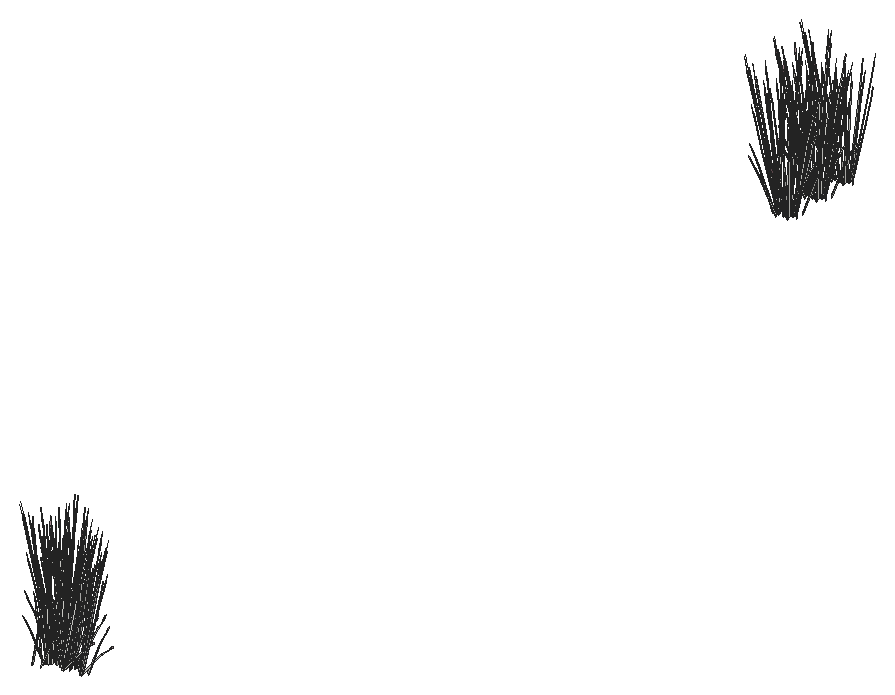
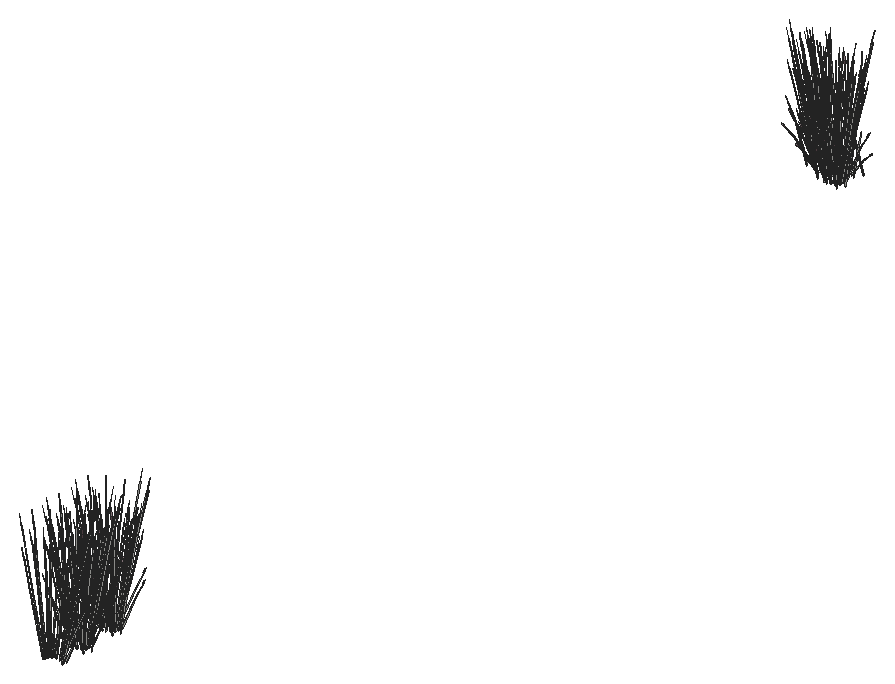
# SketchUp Ruby script. Lengths in inches.
U = 1.inch
M = Sketchup.active_model
def pt(a) = Geom::Point3d.new(a.map { |v| v * U })
def face(e, loops, mat)
  f = e.add_face(loops[0].map { |a| pt(a) })
  loops[1..].each { |l| e.add_face(l.map { |a| pt(a) }).erase! }
  f.material = f.back_material = mat if mat
  f
end
# faces: each face lists its corners as indices into pts; further lists are holes
def faces(e, pts, list, mat = nil) = list.each { |f| face(e, (f[0].is_a?(Array) ? f : [f]).map { |l| l.map { |i| pts[i] } }, mat) }
# xy, xz, yz: faces in a plane at the given z, y or x. An outline is a flat list of corners, or four numbers for a rectangle; further outlines are holes
def ring(l) = l.size == 4 ? [[l[0], l[1]], [l[2], l[1]], [l[2], l[3]], [l[0], l[3]]] : l.each_slice(2).to_a
def flat(e, list, mat, &to3) = list.each { |f| face(e, (f[0].is_a?(Array) ? f : [f]).map { |l| ring(l).map { |u, v| to3.(u, v) } }, mat) }
def xy(e, z, list, mat = nil) = flat(e, list, mat) { |x, y| [x, y, z] }
def xz(e, y, list, mat = nil) = flat(e, list, mat) { |x, z| [x, y, z] }
def yz(e, x, list, mat = nil) = flat(e, list, mat) { |y, z| [x, y, z] }
def lines(e, pts, list) = list.each { |a, b| e.add_line(pt(pts[a]), pt(pts[b])) }
# prism: a flat outline (further loops are holes) pulled along v
def prism(e, loops, v, mat = nil)
  f = face(e, loops, mat); d = Geom::Vector3d.new(v.map { |x| x * U })
  f.pushpull(f.normal.samedirection?(d) ? d.length : -d.length)
end
def box(e, o, s, mat = nil) = prism(e, [[o, [o[0] + s[0], o[1], o[2]], [o[0] + s[0], o[1] + s[1], o[2]], [o[0], o[1] + s[1], o[2]]]], [0, 0, s[2]], mat)
def at(x, y, z, deg = 0) = Geom::Transformation.translation(pt([x, y, z])) * Geom::Transformation.rotation(ORIGIN, Z_AXIS, deg.degrees)
def axes(o, x, y, z) = Geom::Transformation.new([*x, 0, *y, 0, *z, 0, *pt(o).to_a, 1])
def part(name) = M.definitions.add(name)
# library, detail: a bought-in or finely detailed component or shape, given as its bounding box
def library(name, o, s) = part(name).tap { |d| box(d.entities, o, s) }
def detail(e, o, s) = box(e.add_group.entities, o, s)
def put(e, d, t, mat = nil) = e.add_instance(d, t).tap { |i| i.material = mat if mat }
def group(e, t, mat = nil) = e.add_group.tap { |g| g.transformation = t; g.material = mat if mat }.entities
root = M.entities
M.materials.add("LightPink_Translucent").color = [144, 107, 117]
M.materials["LightPink_Translucent"].alpha = 0.75
c1 = part("blade")
p = [[2.15,0.21,22],[0,0.17,0],[0.09,0.45,0],[2.18,0.31,22],[2.29,0.31,22],[0.38,0.45,0],
  [2.48,0.24,33],[2.49,0.24,33],[2.48,0.22,33]]
faces(c1.entities,p,[[0,1,2,3],[4,5,2,3],[6,3,4,7],[8,0,3,6]])
c2 = part("seeds")
p = [[0.3,-0.1,1.38],[-0.01,-0.03,1.59],[-0.01,-0.03,0.03],[0.14,-0.07,-0.07],[0.29,-0.03,3],[0.15,0.01,3.11]]
faces(c2.entities,p,[[0,1,2,3],[1,0,4,5]],"LightPink_Translucent")
c3 = part("blade with seeds")
put(c3.entities,c1,at(0,0,0))
put(c3.entities,c2,axes([2.4,0.25,30.99],[1.5799,-0.05474,1.17369],[-0.12525,1.92788,0.29478],[-0.07173,-0.02425,1.56792]))
put(root,c3,axes([334.01,30.38,52.18],[0.22948,-0.24822,0.05682],[0.32679,0.14452,0.44729],[-0.10565,-0.07958,0.68204]))
put(root,c3,axes([341.83,29.48,52.46],[-0.41962,-0.10901,0.31292],[0.12239,-0.31802,-0.40398],[0.16894,-0.02916,0.77298]))
put(root,c3,axes([337.4375,28.9,52.18],[0.14265,-0.35629,0.42415],[0.46898,0.12183,0.34973],[-0.18443,0.02141,0.87768]))
put(root,c3,axes([331.05,26.46,52.16],[0.05728,-0.02359,1.56736],[0.47345,0.15692,-0.1481],[-0.01113,0.13066,0.27737]))
put(root,c3,axes([335.14,30.62,52.46],[-0.15222,0.30049,0.31292],[-0.44409,-0.08764,-0.40398],[-0.04072,-0.12098,0.77298]))
put(root,c3,axes([337.4,28.8,52.18],[-0.18545,-0.26643,0.05682],[0.33817,-0.13041,0.44729],[-0.14907,0.02573,0.68204]))
put(root,c3,axes([336.28,30.75,52.18],[0.35954,0.26661,0.42415],[-0.38183,0.22994,0.34973],[0.06632,-0.12508,0.87768]))
put(root,c3,axes([334.11,30.36,52.8],[-0.33698,0.3746,-0.12034],[-0.48801,-0.21581,-0.66795],[-0.16964,-0.10584,1.01494]))
put(root,c3,axes([336.41,30.77,52.18],[0.41493,0.01821,0.05682],[-0.01138,0.27493,0.44729],[0.04342,-0.10531,0.68204]))
put(root,c3,axes([338.86,29.54,52.16],[-0.04566,-0.03421,1.56736],[0.09987,-0.36669,-0.1481],[0.17984,-0.02343,0.27737]))
put(root,c3,axes([336.1,30.96,52.46],[-0.34164,0.20573,0.31292],[-0.3234,-0.23491,-0.40398],[0.04921,-0.11936,0.77298]))
put(root,c3,axes([332.92,28.05,52.17],[-0.08245,0.05073,1.54581],[0.00701,0.37067,-0.24447],[-0.18899,0.0482,0.12397]))
put(root,c3,axes([333.14,26.625,52.17],[0.064,0.06292,1.54581],[0.51651,0.02472,-0.24447],[0.05194,0.13877,0.12397]))
put(root,c3,axes([337.2,29.07,52.46],[-0.28729,-0.24465,0.31292],[0.32804,-0.23159,-0.40398],[0.16667,0.03524,0.77298]))
put(root,c3,axes([334.08,30.67,52.46],[0.07798,0.31474,0.31292],[-0.44579,0.08311,-0.40398],[-0.11974,-0.09019,0.77298]))
put(root,c3,axes([342.21,29.58,52.18],[0.18545,0.26643,0.05682],[-0.33817,0.13041,0.44729],[0.14907,-0.02573,0.68204]))
put(root,c3,axes([332.74,30.875,52.5],[0.41698,-0.28837,0.47505],[0.35962,0.30624,0.3917],[-0.19563,-0.05319,0.983]))
put(root,c3,axes([338.07,31.53,52.16],[-0.06595,-0.00297,1.56736],[-0.27386,-0.31799,-0.1481],[0.10998,-0.10455,0.27737]))
put(root,c3,axes([342.18,29.48,52.18],[-0.14265,0.35629,0.42415],[-0.46898,-0.12183,0.34973],[0.18443,-0.02141,0.87768]))
put(root,c3,axes([337.73,28.99,52.17],[0.10831,-0.00661,1.54581],[0.29709,-0.30358,-0.24447],[0.19266,0.04007,0.12397]))
put(root,c3,axes([337.78,28.9,52.46],[0.41962,0.10901,0.31292],[-0.12239,0.31802,-0.40398],[-0.16894,0.02916,0.77298]))
put(root,c3,axes([333.39,28.69,52.18],[-0.12522,-0.35963,0.42415],[0.49122,-0.06241,0.34973],[-0.14477,0.08458,0.87768]))
put(root,c3,axes([333.3,28.62,52.18],[-0.34663,-0.16434,0.05682],[0.20181,-0.23402,0.44729],[-0.11113,0.07566,0.68204]))
put(root,c3,axes([332.93,30.87,52.18],[0.02542,-0.29714,0.05682],[0.38391,0.00815,0.44729],[-0.14706,-0.03109,0.68204]))
put(root,c3,axes([336.69,31.59,52.46],[-0.43951,0.05584,0.31292],[-0.11606,-0.31924,-0.40398],[0.12595,-0.08575,0.77298]))
put(root,c3,axes([343.02,30.64,52.16],[-0.04566,-0.03421,1.56736],[0.09987,-0.36669,-0.1481],[0.17984,-0.02343,0.27737]))
put(root,c3,axes([333.7,28.57,52.46],[0.43951,-0.05584,0.31292],[0.11606,0.31924,-0.40398],[-0.12595,0.08575,0.77298]))
put(root,c3,axes([332,28.43,52.16],[0.06444,0.01048,1.56736],[0.19934,0.34525,-0.1481],[-0.13191,0.09062,0.27737]))
put(root,c3,axes([337.08,29.15,52.17],[-0.08245,0.05073,1.54581],[0.00701,0.37067,-0.24447],[-0.18899,0.0482,0.12397]))
put(root,c3,axes([337.46,29.29,52.18],[-0.02542,0.29714,0.05682],[-0.38391,-0.00815,0.44729],[0.14706,0.03109,0.68204]))
put(root,c3,axes([337.5,29.2,52.18],[-0.3723,0.25748,0.42415],[-0.32109,-0.27343,0.34973],[0.17467,0.04749,0.87768]))
put(root,c3,axes([341.36,30.17,52.46],[-0.28729,-0.24465,0.31292],[0.32804,-0.23159,-0.40398],[0.16667,0.03524,0.77298]))
put(root,c3,axes([337.09,31.54,52.18],[0.34663,0.16434,0.05682],[-0.20181,0.23402,0.44729],[0.11113,-0.07566,0.68204]))
put(root,c3,axes([337,31.47,52.18],[0.12522,0.35963,0.42415],[-0.49122,0.06241,0.34973],[0.14477,-0.08458,0.87768]))
put(root,c3,axes([332.7,29.48,52.99],[0.44556,0.1043,-0.05733],[-0.13706,0.32103,-0.25992],[-0.07288,0.04874,0.85731]))
put(root,c3,axes([336.3125,29.5,52.46],[-0.07798,-0.31474,0.31292],[0.44579,-0.08311,-0.40398],[0.11974,0.09019,0.77298]))
put(root,c3,axes([332.4,30.48,52.16],[0.03743,0.039,1.56736],[-0.18045,0.35054,-0.1481],[-0.18276,0.00254,0.27737]))
put(root,c3,axes([341.88,30.08,52.17],[0.10831,-0.00661,1.54581],[0.29709,-0.30358,-0.24447],[0.19266,0.04007,0.12397]))
put(root,c3,axes([337.55,29.79,52.18],[-0.12522,-0.35963,0.42415],[0.49122,-0.06241,0.34973],[-0.14477,0.08458,0.87768]))
put(root,c3,axes([337.45,29.72,52.18],[-0.34663,-0.16434,0.05682],[0.20181,-0.23402,0.44729],[-0.11113,0.07566,0.68204]))
put(root,c3,axes([333.1875,31.09,52.46],[0.28729,0.24465,0.31292],[-0.32804,0.23159,-0.40398],[-0.16667,-0.03524,0.77298]))
put(root,c3,axes([334.29,29.21,52.46],[0.34164,-0.20573,0.31292],[0.3234,0.23491,-0.40398],[-0.04921,0.11936,0.77298]))
put(root,c3,axes([335.88,29.9375,52.16],[0.00149,-0.04731,1.56736],[0.4327,-0.20872,-0.1481],[0.1503,0.0745,0.27737]))
put(root,c3,axes([337.85,29.67,52.46],[0.43951,-0.05584,0.31292],[0.11606,0.31924,-0.40398],[-0.12595,0.08575,0.77298]))
put(root,c3,axes([333.98,29.39,52.18],[-0.41493,-0.01821,0.05682],[0.01138,-0.27493,0.44729],[-0.04342,0.10531,0.68204]))
put(root,c3,axes([336.16,29.52,52.16],[0.06444,0.01048,1.56736],[0.19934,0.34525,-0.1481],[-0.13191,0.09062,0.27737]))
put(root,c3,axes([334.11,29.42,52.18],[-0.35954,-0.26661,0.42415],[0.38183,-0.22994,0.34973],[-0.06632,0.12508,0.87768]))
put(root,c3,axes([335.25,29.55,52.46],[0.15222,-0.30049,0.31292],[0.44409,0.08764,-0.40398],[0.04072,0.12098,0.77298]))
put(root,c3,axes([341.62,30.39,52.18],[-0.02542,0.29714,0.05682],[-0.38391,-0.00815,0.44729],[0.14706,0.03109,0.68204]))
put(root,c3,axes([341.65,30.29,52.18],[-0.3723,0.25748,0.42415],[-0.32109,-0.27343,0.34973],[0.17467,0.04749,0.87768]))
put(root,c3,axes([336.38,29.78,52.18],[-0.22948,0.24822,0.05682],[-0.32679,-0.14452,0.44729],[0.10565,0.07958,0.68204]))
put(root,c3,axes([335.84,30.62,52.99],[0.34892,-0.22417,-0.05733],[0.3197,0.24551,-0.25992],[0.02251,0.06957,0.85731]))
put(root,c3,axes([336.76,32.36,52.46],[-0.41962,-0.10901,0.31292],[0.12239,-0.31802,-0.40398],[0.16894,-0.02916,0.77298]))
put(root,c3,axes([336.48,29.71,52.18],[-0.5022,0.08967,0.42415],[-0.08716,-0.35177,0.34973],[0.11811,0.10367,0.87768]))
put(root,c3,axes([336.85,30.57,52.99],[0.44556,0.1043,-0.05733],[-0.13706,0.32103,-0.25992],[-0.07288,0.04874,0.85731]))
put(root,c3,axes([332.37,31.78,52.18],[0.14265,-0.35629,0.42415],[0.46898,0.12183,0.34973],[-0.18443,0.02141,0.87768]))
put(root,c3,axes([332.34,31.68,52.18],[-0.18545,-0.26643,0.05682],[0.33817,-0.13041,0.44729],[-0.14907,0.02573,0.68204]))
put(root,c3,axes([340.47,30.59,52.46],[-0.07798,-0.31474,0.31292],[0.44579,-0.08311,-0.40398],[0.11974,0.09019,0.77298]))
put(root,c3,axes([335.11,29.82,52.18],[-0.37205,0.1328,0.05682],[-0.18211,-0.24217,0.44729],[0.03593,0.10675,0.68204]))
put(root,c3,axes([332.93,29.4375,52.17],[-0.01255,0.07733,1.54581],[0.35618,0.269,-0.24447],[-0.09325,0.12721,0.12397]))
put(root,c3,axes([334.07,29.26,52.77],[0.55492,0.01936,-0.11927],[-0.01517,0.36657,-0.66198],[-0.03855,0.14118,1.00587]))
put(root,c3,axes([335.24,29.79,52.47],[-0.49753,-0.10215,0.47081],[0.17013,-0.33585,0.3882],[0.0299,0.13207,0.97422]))
put(root,c3,axes([338.45,30.3,52.46],[0.34164,-0.20573,0.31292],[0.3234,0.23491,-0.40398],[-0.04921,0.11936,0.77298]))
put(root,c3,axes([340.04,31.03,52.16],[0.00149,-0.04731,1.56736],[0.4327,-0.20872,-0.1481],[0.1503,0.0745,0.27737]))
put(root,c3,axes([338.14,30.49,52.18],[-0.41493,-0.01821,0.05682],[0.01138,-0.27493,0.44729],[-0.04342,0.10531,0.68204]))
put(root,c3,axes([338.27,30.51,52.18],[-0.35954,-0.26661,0.42415],[0.38183,-0.22994,0.34973],[-0.06632,0.12508,0.87768]))
put(root,c3,axes([337.14,32.46,52.18],[0.18545,0.26643,0.05682],[-0.33817,0.13041,0.44729],[0.14907,-0.02573,0.68204]))
put(root,c3,axes([339.4,30.64,52.46],[0.15222,-0.30049,0.31292],[0.44409,0.08764,-0.40398],[0.04072,0.12098,0.77298]))
put(root,c3,axes([337.11,32.36,52.18],[-0.14265,0.35629,0.42415],[-0.46898,-0.12183,0.34973],[0.18443,-0.02141,0.87768]))
put(root,c3,axes([332.72,31.78,52.46],[0.41962,0.10901,0.31292],[-0.12239,0.31802,-0.40398],[-0.16894,0.02916,0.77298]))
put(root,c3,axes([332.89,30.23,52.16],[0.05728,-0.02359,1.56736],[0.47345,0.15692,-0.1481],[-0.01113,0.13066,0.27737]))
put(root,c3,axes([340.54,30.875,52.18],[-0.22948,0.24822,0.05682],[-0.32679,-0.14452,0.44729],[0.10565,0.07958,0.68204]))
put(root,c3,axes([340,31.71,52.99],[0.34892,-0.22417,-0.05733],[0.3197,0.24551,-0.25992],[0.02251,0.06957,0.85731]))
put(root,c3,axes([340.64,30.81,52.18],[-0.5022,0.08967,0.42415],[-0.08716,-0.35177,0.34973],[0.11811,0.10367,0.87768]))
put(root,c3,axes([337.95,33.52,52.16],[-0.04566,-0.03421,1.56736],[0.09987,-0.36669,-0.1481],[0.17984,-0.02343,0.27737]))
put(root,c3,axes([339.27,30.91,52.18],[-0.37205,0.1328,0.05682],[-0.18211,-0.24217,0.44729],[0.03593,0.10675,0.68204]))
put(root,c3,axes([337.09,30.53,52.17],[-0.01255,0.07733,1.54581],[0.35618,0.269,-0.24447],[-0.09325,0.12721,0.12397]))
put(root,c3,axes([334.98,30.4,52.17],[0.064,0.06292,1.54581],[0.51651,0.02472,-0.24447],[0.05194,0.13877,0.12397]))
put(root,c3,axes([338.23,30.36,52.77],[0.55492,0.01936,-0.11927],[-0.01517,0.36657,-0.66198],[-0.03855,0.14118,1.00587]))
put(root,c3,axes([339.4,30.89,52.47],[-0.49753,-0.10215,0.47081],[0.17013,-0.33585,0.3882],[0.0299,0.13207,0.97422]))
put(root,c3,axes([336.29,33.04,52.46],[-0.28729,-0.24465,0.31292],[0.32804,-0.23159,-0.40398],[0.16667,0.03524,0.77298]))
put(root,c3,axes([332.48,32.66,52.18],[-0.12522,-0.35963,0.42415],[0.49122,-0.06241,0.34973],[-0.14477,0.08458,0.87768]))
put(root,c3,axes([332.39,32.59,52.18],[-0.34663,-0.16434,0.05682],[0.20181,-0.23402,0.44729],[-0.11113,0.07566,0.68204]))
put(root,c3,axes([337.05,31.33,52.16],[0.05728,-0.02359,1.56736],[0.47345,0.15692,-0.1481],[-0.01113,0.13066,0.27737]))
put(root,c3,axes([332.79,32.54,52.46],[0.43951,-0.05584,0.31292],[0.11606,0.31924,-0.40398],[-0.12595,0.08575,0.77298]))
put(root,c3,axes([339.14,31.49,52.17],[0.064,0.06292,1.54581],[0.51651,0.02472,-0.24447],[0.05194,0.13877,0.12397]))
put(root,c3,axes([331.09,32.4,52.16],[0.06444,0.01048,1.56736],[0.19934,0.34525,-0.1481],[-0.13191,0.09062,0.27737]))
put(root,c3,axes([336.55,33.27,52.18],[-0.02542,0.29714,0.05682],[-0.38391,-0.00815,0.44729],[0.14706,0.03109,0.68204]))
put(root,c3,axes([336.59,33.17,52.18],[-0.3723,0.25748,0.42415],[-0.32109,-0.27343,0.34973],[0.17467,0.04749,0.87768]))
put(root,c3,axes([331.79,33.45,52.99],[0.44556,0.1043,-0.05733],[-0.13706,0.32103,-0.25992],[-0.07288,0.04874,0.85731]))
put(root,c3,axes([335.4,33.47,52.46],[-0.07798,-0.31474,0.31292],[0.44579,-0.08311,-0.40398],[0.11974,0.09019,0.77298]))
put(root,c3,axes([333.38,33.18,52.46],[0.34164,-0.20573,0.31292],[0.3234,0.23491,-0.40398],[-0.04921,0.11936,0.77298]))
put(root,c3,axes([334.97,33.91,52.16],[0.00149,-0.04731,1.56736],[0.4327,-0.20872,-0.1481],[0.1503,0.0745,0.27737]))
put(root,c3,axes([333.07,33.37,52.18],[-0.41493,-0.01821,0.05682],[0.01138,-0.27493,0.44729],[-0.04342,0.10531,0.68204]))
put(root,c3,axes([333.2,33.39,52.18],[-0.35954,-0.26661,0.42415],[0.38183,-0.22994,0.34973],[-0.06632,0.12508,0.87768]))
put(root,c3,axes([334.34,33.52,52.46],[0.15222,-0.30049,0.31292],[0.44409,0.08764,-0.40398],[0.04072,0.12098,0.77298]))
put(root,c3,axes([335.47,33.75,52.18],[-0.22948,0.24822,0.05682],[-0.32679,-0.14452,0.44729],[0.10565,0.07958,0.68204]))
put(root,c3,axes([334.94,34.59,52.99],[0.34892,-0.22417,-0.05733],[0.3197,0.24551,-0.25992],[0.02251,0.06957,0.85731]))
put(root,c3,axes([335.57,33.68,52.18],[-0.5022,0.08967,0.42415],[-0.08716,-0.35177,0.34973],[0.11811,0.10367,0.87768]))
put(root,c3,axes([334.2,33.79,52.18],[-0.37205,0.1328,0.05682],[-0.18211,-0.24217,0.44729],[0.03593,0.10675,0.68204]))
put(root,c3,axes([333.16,33.24,52.77],[0.55492,0.01936,-0.11927],[-0.01517,0.36657,-0.66198],[-0.03855,0.14118,1.00587]))
put(root,c3,axes([334.33,33.77,52.47],[-0.49753,-0.10215,0.47081],[0.17013,-0.33585,0.3882],[0.0299,0.13207,0.97422]))
put(root,c3,axes([331.98,34.2,52.16],[0.05728,-0.02359,1.56736],[0.47345,0.15692,-0.1481],[-0.01113,0.13066,0.27737]))
put(root,c3,axes([335.78,274.7,52.16],[-0.05128,0.02985,1.56736],[-0.5024,-0.1007,-0.1481],[-0.01819,-0.13025,0.27737]))
put(root,c3,axes([333.05,274.125,52.16],[-0.00942,0.04684,1.56736],[-0.46458,0.16998,-0.1481],[-0.13671,-0.08689,0.27737]))
put(root,c3,axes([332.94,274.96,52.5],[0.56246,-0.10044,0.47505],[0.09762,0.39398,0.3917],[-0.13228,-0.11611,0.983]))
put(root,c3,axes([334.22,275.03,52.18],[0.49753,0.10215,0.42415],[-0.17013,0.33585,0.34973],[-0.0299,-0.13207,0.87768]))
put(root,c3,axes([334.35,275,52.18],[0.37205,-0.1328,0.05682],[0.18211,0.24217,0.44729],[-0.03593,-0.10675,0.68204]))
put(root,c3,axes([333.07,275.04,52.18],[0.22948,-0.24822,0.05682],[0.32679,0.14452,0.44729],[-0.10565,-0.07958,0.68204]))
put(root,c3,axes([334.21,275.28,52.46],[-0.15222,0.30049,0.31292],[-0.44409,-0.08764,-0.40398],[-0.04072,-0.12098,0.77298]))
put(root,c3,axes([335.34,275.4,52.18],[0.35954,0.26661,0.42415],[-0.38183,0.22994,0.34973],[0.06632,-0.12508,0.87768]))
put(root,c3,axes([333.18,275.02,52.8],[-0.33698,0.3746,-0.12034],[-0.48801,-0.21581,-0.66795],[-0.16964,-0.10584,1.01494]))
put(root,c3,axes([335.48,275.43,52.18],[0.41493,0.01821,0.05682],[-0.01138,0.27493,0.44729],[0.04342,-0.10531,0.68204]))
put(root,c3,axes([335.17,275.62,52.46],[-0.34164,0.20573,0.31292],[-0.3234,-0.23491,-0.40398],[0.04921,-0.11936,0.77298]))
put(root,c3,axes([333.14,275.33,52.46],[0.07798,0.31474,0.31292],[-0.44579,0.08311,-0.40398],[-0.11974,-0.09019,0.77298]))
put(root,c3,axes([331.8,275.53,52.5],[0.41698,-0.28837,0.47505],[0.35962,0.30624,0.3917],[-0.19563,-0.05319,0.983]))
put(root,c3,axes([337.14,276.1875,52.16],[-0.06595,-0.00297,1.56736],[-0.27386,-0.31799,-0.1481],[0.10998,-0.10455,0.27737]))
put(root,c3,axes([331.99,275.53,52.18],[0.02542,-0.29714,0.05682],[0.38391,0.00815,0.44729],[-0.14706,-0.03109,0.68204]))
put(root,c3,axes([335.76,276.25,52.46],[-0.43951,0.05584,0.31292],[-0.11606,-0.31924,-0.40398],[0.12595,-0.08575,0.77298]))
put(root,c3,axes([336.16,276.2,52.18],[0.34663,0.16434,0.05682],[-0.20181,0.23402,0.44729],[0.11113,-0.07566,0.68204]))
put(root,c3,axes([336.0625,276.13,52.18],[0.12522,0.35963,0.42415],[-0.49122,0.06241,0.34973],[0.14477,-0.08458,0.87768]))
put(root,c3,axes([331.47,275.14,52.16],[0.03743,0.039,1.56736],[-0.18045,0.35054,-0.1481],[-0.18276,0.00254,0.27737]))
put(root,c3,axes([332.25,275.75,52.46],[0.28729,0.24465,0.31292],[-0.32804,0.23159,-0.40398],[-0.16667,-0.03524,0.77298]))
put(root,c3,axes([335.83,277.01,52.46],[-0.41962,-0.10901,0.31292],[0.12239,-0.31802,-0.40398],[0.16894,-0.02916,0.77298]))
put(root,c3,axes([331.4375,276.43,52.18],[0.14265,-0.35629,0.42415],[0.46898,0.12183,0.34973],[-0.18443,0.02141,0.87768]))
put(root,c3,axes([331.4,276.34,52.18],[-0.18545,-0.26643,0.05682],[0.33817,-0.13041,0.44729],[-0.14907,0.02573,0.68204]))
put(root,c3,axes([336.21,277.11,52.18],[0.18545,0.26643,0.05682],[-0.33817,0.13041,0.44729],[0.14907,-0.02573,0.68204]))
put(root,c3,axes([336.18,277.02,52.18],[-0.14265,0.35629,0.42415],[-0.46898,-0.12183,0.34973],[0.18443,-0.02141,0.87768]))
put(root,c3,axes([331.78,276.4375,52.46],[0.41962,0.10901,0.31292],[-0.12239,0.31802,-0.40398],[-0.16894,0.02916,0.77298]))
put(root,c3,axes([337.02,278.17,52.16],[-0.04566,-0.03421,1.56736],[0.09987,-0.36669,-0.1481],[0.17984,-0.02343,0.27737]))
put(root,c3,axes([335.36,277.7,52.46],[-0.28729,-0.24465,0.31292],[0.32804,-0.23159,-0.40398],[0.16667,0.03524,0.77298]))
put(root,c3,axes([331.55,277.32,52.18],[-0.12522,-0.35963,0.42415],[0.49122,-0.06241,0.34973],[-0.14477,0.08458,0.87768]))
put(root,c3,axes([331.45,277.25,52.18],[-0.34663,-0.16434,0.05682],[0.20181,-0.23402,0.44729],[-0.11113,0.07566,0.68204]))
put(root,c3,axes([331.85,277.2,52.46],[0.43951,-0.05584,0.31292],[0.11606,0.31924,-0.40398],[-0.12595,0.08575,0.77298]))
put(root,c3,axes([330.16,277.06,52.16],[0.06444,0.01048,1.56736],[0.19934,0.34525,-0.1481],[-0.13191,0.09062,0.27737]))
put(root,c3,axes([335.62,277.92,52.18],[-0.02542,0.29714,0.05682],[-0.38391,-0.00815,0.44729],[0.14706,0.03109,0.68204]))
put(root,c3,axes([335.65,277.83,52.18],[-0.3723,0.25748,0.42415],[-0.32109,-0.27343,0.34973],[0.17467,0.04749,0.87768]))
put(root,c3,axes([330.85,278.11,52.99],[0.44556,0.1043,-0.05733],[-0.13706,0.32103,-0.25992],[-0.07288,0.04874,0.85731]))
put(root,c3,axes([334.47,278.125,52.46],[-0.07798,-0.31474,0.31292],[0.44579,-0.08311,-0.40398],[0.11974,0.09019,0.77298]))
put(root,c3,axes([332.45,277.84,52.46],[0.34164,-0.20573,0.31292],[0.3234,0.23491,-0.40398],[-0.04921,0.11936,0.77298]))
put(root,c3,axes([334.04,278.57,52.16],[0.00149,-0.04731,1.56736],[0.4327,-0.20872,-0.1481],[0.1503,0.0745,0.27737]))
put(root,c3,axes([332.14,278.02,52.18],[-0.41493,-0.01821,0.05682],[0.01138,-0.27493,0.44729],[-0.04342,0.10531,0.68204]))
put(root,c3,axes([332.27,278.05,52.18],[-0.35954,-0.26661,0.42415],[0.38183,-0.22994,0.34973],[-0.06632,0.12508,0.87768]))
put(root,c3,axes([333.4,278.18,52.46],[0.15222,-0.30049,0.31292],[0.44409,0.08764,-0.40398],[0.04072,0.12098,0.77298]))
put(root,c3,axes([334.54,278.41,52.18],[-0.22948,0.24822,0.05682],[-0.32679,-0.14452,0.44729],[0.10565,0.07958,0.68204]))
put(root,c3,axes([334,279.25,52.99],[0.34892,-0.22417,-0.05733],[0.3197,0.24551,-0.25992],[0.02251,0.06957,0.85731]))
put(root,c3,axes([334.64,278.34,52.18],[-0.5022,0.08967,0.42415],[-0.08716,-0.35177,0.34973],[0.11811,0.10367,0.87768]))
put(root,c3,axes([333.27,278.45,52.18],[-0.37205,0.1328,0.05682],[-0.18211,-0.24217,0.44729],[0.03593,0.10675,0.68204]))
put(root,c3,axes([332.23,277.89,52.77],[0.55492,0.01936,-0.11927],[-0.01517,0.36657,-0.66198],[-0.03855,0.14118,1.00587]))
put(root,c3,axes([333.4,278.42,52.47],[-0.49753,-0.10215,0.47081],[0.17013,-0.33585,0.3882],[0.0299,0.13207,0.97422]))
put(root,c3,axes([331.05,278.86,52.16],[0.05728,-0.02359,1.56736],[0.47345,0.15692,-0.1481],[-0.01113,0.13066,0.27737]))
put(root,c3,axes([335.78,284.5,52.16],[-0.05128,0.02985,1.56736],[-0.5024,-0.1007,-0.1481],[-0.01819,-0.13025,0.27737]))
put(root,c3,axes([333.05,283.93,52.16],[-0.00942,0.04684,1.56736],[-0.46458,0.16998,-0.1481],[-0.13671,-0.08689,0.27737]))
put(root,c3,axes([332.94,284.76,52.5],[0.56246,-0.10044,0.47505],[0.09762,0.39398,0.3917],[-0.13228,-0.11611,0.983]))
put(root,c3,axes([334.22,284.83,52.18],[0.49753,0.10215,0.42415],[-0.17013,0.33585,0.34973],[-0.0299,-0.13207,0.87768]))
put(root,c3,axes([334.35,284.81,52.18],[0.37205,-0.1328,0.05682],[0.18211,0.24217,0.44729],[-0.03593,-0.10675,0.68204]))
put(root,c3,axes([333.07,284.84,52.18],[0.22948,-0.24822,0.05682],[0.32679,0.14452,0.44729],[-0.10565,-0.07958,0.68204]))
put(root,c3,axes([334.21,285.08,52.46],[-0.15222,0.30049,0.31292],[-0.44409,-0.08764,-0.40398],[-0.04072,-0.12098,0.77298]))
put(root,c3,axes([335.34,285.21,52.18],[0.35954,0.26661,0.42415],[-0.38183,0.22994,0.34973],[0.06632,-0.12508,0.87768]))
put(root,c3,axes([333.18,284.82,52.8],[-0.33698,0.3746,-0.12034],[-0.48801,-0.21581,-0.66795],[-0.16964,-0.10584,1.01494]))
put(root,c3,axes([335.48,285.23,52.18],[0.41493,0.01821,0.05682],[-0.01138,0.27493,0.44729],[0.04342,-0.10531,0.68204]))
put(root,c3,axes([335.17,285.42,52.46],[-0.34164,0.20573,0.31292],[-0.3234,-0.23491,-0.40398],[0.04921,-0.11936,0.77298]))
put(root,c3,axes([333.14,285.13,52.46],[0.07798,0.31474,0.31292],[-0.44579,0.08311,-0.40398],[-0.11974,-0.09019,0.77298]))
put(root,c3,axes([331.8,285.33,52.5],[0.41698,-0.28837,0.47505],[0.35962,0.30624,0.3917],[-0.19563,-0.05319,0.983]))
put(root,c3,axes([337.14,285.99,52.16],[-0.06595,-0.00297,1.56736],[-0.27386,-0.31799,-0.1481],[0.10998,-0.10455,0.27737]))
put(root,c3,axes([331.99,285.33,52.18],[0.02542,-0.29714,0.05682],[0.38391,0.00815,0.44729],[-0.14706,-0.03109,0.68204]))
put(root,c3,axes([335.76,286.05,52.46],[-0.43951,0.05584,0.31292],[-0.11606,-0.31924,-0.40398],[0.12595,-0.08575,0.77298]))
put(root,c3,axes([336.16,286,52.18],[0.34663,0.16434,0.05682],[-0.20181,0.23402,0.44729],[0.11113,-0.07566,0.68204]))
put(root,c3,axes([336.0625,285.93,52.18],[0.12522,0.35963,0.42415],[-0.49122,0.06241,0.34973],[0.14477,-0.08458,0.87768]))
put(root,c3,axes([331.47,284.94,52.16],[0.03743,0.039,1.56736],[-0.18045,0.35054,-0.1481],[-0.18276,0.00254,0.27737]))
put(root,c3,axes([332.25,285.55,52.46],[0.28729,0.24465,0.31292],[-0.32804,0.23159,-0.40398],[-0.16667,-0.03524,0.77298]))
put(root,c3,axes([335.83,286.82,52.46],[-0.41962,-0.10901,0.31292],[0.12239,-0.31802,-0.40398],[0.16894,-0.02916,0.77298]))
put(root,c3,axes([331.4375,286.24,52.18],[0.14265,-0.35629,0.42415],[0.46898,0.12183,0.34973],[-0.18443,0.02141,0.87768]))
put(root,c3,axes([331.4,286.14,52.18],[-0.18545,-0.26643,0.05682],[0.33817,-0.13041,0.44729],[-0.14907,0.02573,0.68204]))
put(root,c3,axes([336.21,286.92,52.18],[0.18545,0.26643,0.05682],[-0.33817,0.13041,0.44729],[0.14907,-0.02573,0.68204]))
put(root,c3,axes([336.18,286.82,52.18],[-0.14265,0.35629,0.42415],[-0.46898,-0.12183,0.34973],[0.18443,-0.02141,0.87768]))
put(root,c3,axes([331.78,286.24,52.46],[0.41962,0.10901,0.31292],[-0.12239,0.31802,-0.40398],[-0.16894,0.02916,0.77298]))
put(root,c3,axes([337.02,287.97,52.16],[-0.04566,-0.03421,1.56736],[0.09987,-0.36669,-0.1481],[0.17984,-0.02343,0.27737]))
put(root,c3,axes([335.36,287.5,52.46],[-0.28729,-0.24465,0.31292],[0.32804,-0.23159,-0.40398],[0.16667,0.03524,0.77298]))
put(root,c3,axes([331.55,287.125,52.18],[-0.12522,-0.35963,0.42415],[0.49122,-0.06241,0.34973],[-0.14477,0.08458,0.87768]))
put(root,c3,axes([331.45,287.05,52.18],[-0.34663,-0.16434,0.05682],[0.20181,-0.23402,0.44729],[-0.11113,0.07566,0.68204]))
put(root,c3,axes([331.85,287,52.46],[0.43951,-0.05584,0.31292],[0.11606,0.31924,-0.40398],[-0.12595,0.08575,0.77298]))
put(root,c3,axes([330.16,286.86,52.16],[0.06444,0.01048,1.56736],[0.19934,0.34525,-0.1481],[-0.13191,0.09062,0.27737]))
put(root,c3,axes([335.62,287.72,52.18],[-0.02542,0.29714,0.05682],[-0.38391,-0.00815,0.44729],[0.14706,0.03109,0.68204]))
put(root,c3,axes([335.65,287.63,52.18],[-0.3723,0.25748,0.42415],[-0.32109,-0.27343,0.34973],[0.17467,0.04749,0.87768]))
put(root,c3,axes([330.85,287.91,52.99],[0.44556,0.1043,-0.05733],[-0.13706,0.32103,-0.25992],[-0.07288,0.04874,0.85731]))
put(root,c3,axes([334.47,287.93,52.46],[-0.07798,-0.31474,0.31292],[0.44579,-0.08311,-0.40398],[0.11974,0.09019,0.77298]))
put(root,c3,axes([332.45,287.64,52.46],[0.34164,-0.20573,0.31292],[0.3234,0.23491,-0.40398],[-0.04921,0.11936,0.77298]))
put(root,c3,axes([334.04,288.37,52.16],[0.00149,-0.04731,1.56736],[0.4327,-0.20872,-0.1481],[0.1503,0.0745,0.27737]))
put(root,c3,axes([332.14,287.83,52.18],[-0.41493,-0.01821,0.05682],[0.01138,-0.27493,0.44729],[-0.04342,0.10531,0.68204]))
put(root,c3,axes([332.27,287.85,52.18],[-0.35954,-0.26661,0.42415],[0.38183,-0.22994,0.34973],[-0.06632,0.12508,0.87768]))
put(root,c3,axes([333.4,287.98,52.46],[0.15222,-0.30049,0.31292],[0.44409,0.08764,-0.40398],[0.04072,0.12098,0.77298]))
put(root,c3,axes([334.54,288.21,52.18],[-0.22948,0.24822,0.05682],[-0.32679,-0.14452,0.44729],[0.10565,0.07958,0.68204]))
put(root,c3,axes([334,289.05,52.99],[0.34892,-0.22417,-0.05733],[0.3197,0.24551,-0.25992],[0.02251,0.06957,0.85731]))
put(root,c3,axes([334.64,288.14,52.18],[-0.5022,0.08967,0.42415],[-0.08716,-0.35177,0.34973],[0.11811,0.10367,0.87768]))
put(root,c3,axes([333.27,288.25,52.18],[-0.37205,0.1328,0.05682],[-0.18211,-0.24217,0.44729],[0.03593,0.10675,0.68204]))
put(root,c3,axes([332.23,287.7,52.77],[0.55492,0.01936,-0.11927],[-0.01517,0.36657,-0.66198],[-0.03855,0.14118,1.00587]))
put(root,c3,axes([333.4,288.22,52.47],[-0.49753,-0.10215,0.47081],[0.17013,-0.33585,0.3882],[0.0299,0.13207,0.97422]))
put(root,c3,axes([331.05,288.66,52.16],[0.05728,-0.02359,1.56736],[0.47345,0.15692,-0.1481],[-0.01113,0.13066,0.27737]))
put(root,c3,axes([335.78,293.48,52.16],[-0.05128,0.02985,1.56736],[-0.5024,-0.1007,-0.1481],[-0.01819,-0.13025,0.27737]))
put(root,c3,axes([333.05,292.9,52.16],[-0.00942,0.04684,1.56736],[-0.46458,0.16998,-0.1481],[-0.13671,-0.08689,0.27737]))
put(root,c3,axes([332.94,293.74,52.5],[0.56246,-0.10044,0.47505],[0.09762,0.39398,0.3917],[-0.13228,-0.11611,0.983]))
put(root,c3,axes([334.22,293.81,52.18],[0.49753,0.10215,0.42415],[-0.17013,0.33585,0.34973],[-0.0299,-0.13207,0.87768]))
put(root,c3,axes([334.35,293.78,52.18],[0.37205,-0.1328,0.05682],[0.18211,0.24217,0.44729],[-0.03593,-0.10675,0.68204]))
put(root,c3,axes([333.07,293.82,52.18],[0.22948,-0.24822,0.05682],[0.32679,0.14452,0.44729],[-0.10565,-0.07958,0.68204]))
put(root,c3,axes([334.21,294.06,52.46],[-0.15222,0.30049,0.31292],[-0.44409,-0.08764,-0.40398],[-0.04072,-0.12098,0.77298]))
put(root,c3,axes([335.34,294.18,52.18],[0.35954,0.26661,0.42415],[-0.38183,0.22994,0.34973],[0.06632,-0.12508,0.87768]))
put(root,c3,axes([333.18,293.79,52.8],[-0.33698,0.3746,-0.12034],[-0.48801,-0.21581,-0.66795],[-0.16964,-0.10584,1.01494]))
put(root,c3,axes([335.48,294.21,52.18],[0.41493,0.01821,0.05682],[-0.01138,0.27493,0.44729],[0.04342,-0.10531,0.68204]))
put(root,c3,axes([335.17,294.39,52.46],[-0.34164,0.20573,0.31292],[-0.3234,-0.23491,-0.40398],[0.04921,-0.11936,0.77298]))
put(root,c3,axes([333.14,294.11,52.46],[0.07798,0.31474,0.31292],[-0.44579,0.08311,-0.40398],[-0.11974,-0.09019,0.77298]))
put(root,c3,axes([331.8,294.3125,52.5],[0.41698,-0.28837,0.47505],[0.35962,0.30624,0.3917],[-0.19563,-0.05319,0.983]))
put(root,c3,axes([337.14,294.97,52.16],[-0.06595,-0.00297,1.56736],[-0.27386,-0.31799,-0.1481],[0.10998,-0.10455,0.27737]))
put(root,c3,axes([331.99,294.31,52.18],[0.02542,-0.29714,0.05682],[0.38391,0.00815,0.44729],[-0.14706,-0.03109,0.68204]))
put(root,c3,axes([335.76,295.03,52.46],[-0.43951,0.05584,0.31292],[-0.11606,-0.31924,-0.40398],[0.12595,-0.08575,0.77298]))
put(root,c3,axes([336.16,294.98,52.18],[0.34663,0.16434,0.05682],[-0.20181,0.23402,0.44729],[0.11113,-0.07566,0.68204]))
put(root,c3,axes([336.0625,294.91,52.18],[0.12522,0.35963,0.42415],[-0.49122,0.06241,0.34973],[0.14477,-0.08458,0.87768]))
put(root,c3,axes([331.47,293.92,52.16],[0.03743,0.039,1.56736],[-0.18045,0.35054,-0.1481],[-0.18276,0.00254,0.27737]))
put(root,c3,axes([332.25,294.53,52.46],[0.28729,0.24465,0.31292],[-0.32804,0.23159,-0.40398],[-0.16667,-0.03524,0.77298]))
put(root,c3,axes([335.83,295.79,52.46],[-0.41962,-0.10901,0.31292],[0.12239,-0.31802,-0.40398],[0.16894,-0.02916,0.77298]))
put(root,c3,axes([331.4375,295.21,52.18],[0.14265,-0.35629,0.42415],[0.46898,0.12183,0.34973],[-0.18443,0.02141,0.87768]))
put(root,c3,axes([331.4,295.12,52.18],[-0.18545,-0.26643,0.05682],[0.33817,-0.13041,0.44729],[-0.14907,0.02573,0.68204]))
put(root,c3,axes([336.21,295.89,52.18],[0.18545,0.26643,0.05682],[-0.33817,0.13041,0.44729],[0.14907,-0.02573,0.68204]))
put(root,c3,axes([336.18,295.8,52.18],[-0.14265,0.35629,0.42415],[-0.46898,-0.12183,0.34973],[0.18443,-0.02141,0.87768]))
